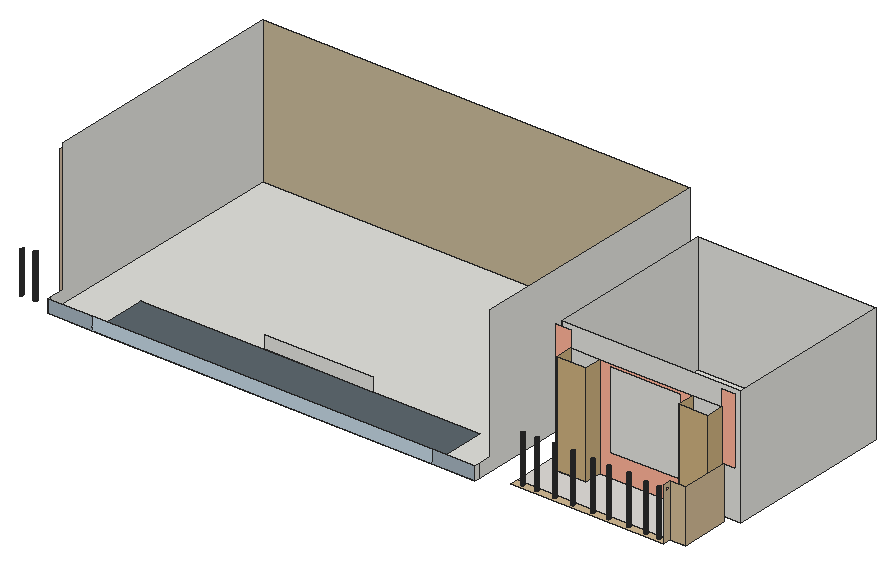
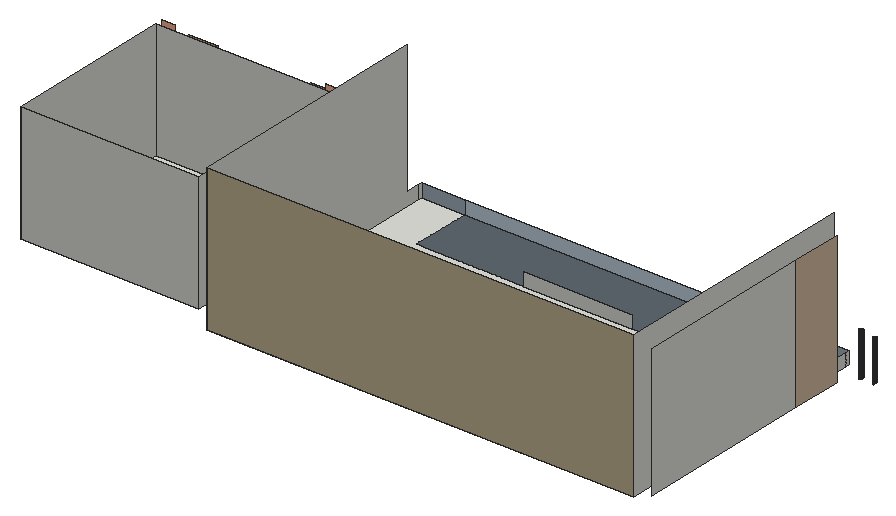
# SketchUp Ruby script. Lengths in inches.
U = 1.inch
M = Sketchup.active_model
def pt(a) = Geom::Point3d.new(a.map { |v| v * U })
def face(e, loops, mat)
  f = e.add_face(loops[0].map { |a| pt(a) })
  loops[1..].each { |l| e.add_face(l.map { |a| pt(a) }).erase! }
  f.material = f.back_material = mat if mat
  f
end
# faces: each face lists its corners as indices into pts; further lists are holes
def faces(e, pts, list, mat = nil) = list.each { |f| face(e, (f[0].is_a?(Array) ? f : [f]).map { |l| l.map { |i| pts[i] } }, mat) }
# xy, xz, yz: faces in a plane at the given z, y or x. An outline is a flat list of corners, or four numbers for a rectangle; further outlines are holes
def ring(l) = l.size == 4 ? [[l[0], l[1]], [l[2], l[1]], [l[2], l[3]], [l[0], l[3]]] : l.each_slice(2).to_a
def flat(e, list, mat, &to3) = list.each { |f| face(e, (f[0].is_a?(Array) ? f : [f]).map { |l| ring(l).map { |u, v| to3.(u, v) } }, mat) }
def xy(e, z, list, mat = nil) = flat(e, list, mat) { |x, y| [x, y, z] }
def xz(e, y, list, mat = nil) = flat(e, list, mat) { |x, z| [x, y, z] }
def yz(e, x, list, mat = nil) = flat(e, list, mat) { |y, z| [x, y, z] }
def lines(e, pts, list) = list.each { |a, b| e.add_line(pt(pts[a]), pt(pts[b])) }
# prism: a flat outline (further loops are holes) pulled along v
def prism(e, loops, v, mat = nil)
  f = face(e, loops, mat); d = Geom::Vector3d.new(v.map { |x| x * U })
  f.pushpull(f.normal.samedirection?(d) ? d.length : -d.length)
end
def box(e, o, s, mat = nil) = prism(e, [[o, [o[0] + s[0], o[1], o[2]], [o[0] + s[0], o[1] + s[1], o[2]], [o[0], o[1] + s[1], o[2]]]], [0, 0, s[2]], mat)
def at(x, y, z, deg = 0) = Geom::Transformation.translation(pt([x, y, z])) * Geom::Transformation.rotation(ORIGIN, Z_AXIS, deg.degrees)
def axes(o, x, y, z) = Geom::Transformation.new([*x, 0, *y, 0, *z, 0, *pt(o).to_a, 1])
def part(name) = M.definitions.add(name)
# library, detail: a bought-in or finely detailed component or shape, given as its bounding box
def library(name, o, s) = part(name).tap { |d| box(d.entities, o, s) }
def detail(e, o, s) = box(e.add_group.entities, o, s)
def put(e, d, t, mat = nil) = e.add_instance(d, t).tap { |i| i.material = mat if mat }
def group(e, t, mat = nil) = e.add_group.tap { |g| g.transformation = t; g.material = mat if mat }.entities
root = M.entities
M.materials.add("[Color B02]").color = [255, 178, 153]
M.materials.add("[Formica Beige]").color = [211, 187, 149]
M.materials.add("[Formica Laminate Dark]").color = [50, 53, 60]
M.materials.add("[Formica Laminate Light]").color = [213, 189, 164]
M.materials.add("[Formica Speckled Grey]").color = [94, 105, 111]
M.materials.add("[Quartz Light Brown]").color = [199, 184, 152]
M.materials.add("[Terrazzo Light Blue]1").color = [165, 180, 191]
M.materials.add("[Terrazzo Light Blue]2").color = [196, 214, 227]
M.materials.add("[Terrazzo Tile Accent]").color = [224, 221, 217]
M.materials.add("[Wood Floor Light]").color = [204, 176, 127]
xy(root,381,[[198.57,119.07,198.57,364.125,588.3,364.125,588.3,119.07,549.2,119.07,549.2,174.4375,238.58,174.4375,238.58,119.07],[179.57,126.78,179.17,126.87,178.8125,127.0625,178.51,127.34,178.3,127.6875,178.18,128.08,178.17,128.48,178.26,128.88,178.45,129.24,178.73,129.54,179.07,129.76,179.46,129.875,179.87,129.89,180.27,129.8,180.63,129.6,180.93,129.33,181.14,128.98,181.26,128.59,181.28,128.18,181.18,127.78,180.99,127.42,180.71,127.125,180.37,126.91,179.98,126.79],[618.46,134.27,618.09,134.32,617.75,134.46,617.45,134.6875,617.22,134.99,617.08,135.33,617.03,135.7,617.08,136.08,617.22,136.42,617.45,136.72,617.75,136.95,618.09,137.09,618.46,137.14,618.84,137.09,619.18,136.95,619.48,136.72,619.71,136.42,619.85,136.08,619.9,135.7,619.85,135.33,619.71,134.99,619.48,134.6875,619.18,134.46,618.84,134.32],[631.71,134.27,631.34,134.32,631,134.46,630.7,134.6875,630.47,134.99,630.33,135.33,630.28,135.7,630.33,136.08,630.47,136.42,630.7,136.72,631,136.95,631.34,137.09,631.71,137.14,632.09,137.09,632.43,136.95,632.73,136.72,632.96,136.42,633.1,136.08,633.15,135.7,633.1,135.33,632.96,134.99,632.73,134.6875,632.43,134.46,632.09,134.32],[647.4,134.27,647.03,134.32,646.68,134.46,646.39,134.6875,646.16,134.99,646.01,135.33,645.96,135.7,646.01,136.08,646.16,136.42,646.39,136.72,646.68,136.95,647.03,137.09,647.4,137.14,647.77,137.09,648.12,136.95,648.42,136.72,648.65,136.42,648.79,136.08,648.84,135.7,648.79,135.33,648.65,134.99,648.42,134.6875,648.12,134.46,647.77,134.32],
  [664.53,134.27,664.16,134.32,663.81,134.46,663.51,134.6875,663.28,134.99,663.14,135.33,663.09,135.7,663.14,136.08,663.28,136.42,663.51,136.72,663.81,136.95,664.16,137.09,664.53,137.14,664.9,137.09,665.25,136.95,665.54,136.72,665.77,136.42,665.92,136.08,665.96,135.7,665.92,135.33,665.77,134.99,665.54,134.6875,665.25,134.46,664.9,134.32],[682.4,134.27,682.03,134.32,681.68,134.46,681.39,134.6875,681.16,134.99,681.01,135.33,680.96,135.7,681.01,136.08,681.16,136.42,681.39,136.72,681.68,136.95,682.03,137.09,682.4,137.14,682.77,137.09,683.12,136.95,683.42,136.72,683.65,136.42,683.79,136.08,683.84,135.7,683.79,135.33,683.65,134.99,683.42,134.6875,683.12,134.46,682.77,134.32],[697.03,134.27,696.66,134.32,696.31,134.46,696.01,134.6875,695.78,134.99,695.64,135.33,695.59,135.7,695.64,136.08,695.78,136.42,696.01,136.72,696.31,136.95,696.66,137.09,697.03,137.14,697.4,137.09,697.75,136.95,698.04,136.72,698.27,136.42,698.42,136.08,698.46,135.7,698.42,135.33,698.27,134.99,698.04,134.6875,697.75,134.46,697.4,134.32],[715.03,134.27,714.66,134.32,714.31,134.46,714.01,134.6875,713.78,134.99,713.64,135.33,713.59,135.7,713.64,136.08,713.78,136.42,714.01,136.72,714.31,136.95,714.66,137.09,715.03,137.14,715.4,137.09,715.75,136.95,716.04,136.72,716.27,136.42,716.42,136.08,716.46,135.7,716.42,135.33,716.27,134.99,716.04,134.6875,715.75,134.46,715.4,134.32],[730.9,134.27,730.53,134.32,730.18,134.46,729.89,134.6875,729.66,134.99,729.51,135.33,729.46,135.7,729.51,136.08,729.66,136.42,729.89,136.72,730.18,136.95,730.53,137.09,730.9,137.14,731.27,137.09,731.62,136.95,731.92,136.72,732.15,136.42,732.29,136.08,732.34,135.7,732.29,135.33,732.15,134.99,731.92,134.6875,731.62,134.46,731.27,134.32],
  [742.96,134.27,742.59,134.32,742.25,134.46,741.95,134.6875,741.72,134.99,741.58,135.33,741.53,135.7,741.58,136.08,741.72,136.42,741.95,136.72,742.25,136.95,742.59,137.09,742.96,137.14,743.34,137.09,743.68,136.95,743.98,136.72,744.21,136.42,744.35,136.08,744.4,135.7,744.35,135.33,744.21,134.99,743.98,134.6875,743.68,134.46,743.34,134.32],[624.7,167.26,651.04,182.57],[735.89,167.26,762.23,182.57],[611.125,189.24,774.15,344.36]])
xy(root,381,[[[611.125,131.74,750.32,138.95],[742.96,134.27,742.59,134.32,742.25,134.46,741.95,134.6875,741.72,134.99,741.58,135.33,741.53,135.7,741.58,136.08,741.72,136.42,741.95,136.72,742.25,136.95,742.59,137.09,742.96,137.14,743.34,137.09,743.68,136.95,743.98,136.72,744.21,136.42,744.35,136.08,744.4,135.7,744.35,135.33,744.21,134.99,743.98,134.6875,743.68,134.46,743.34,134.32],[618.46,134.27,618.09,134.32,617.75,134.46,617.45,134.6875,617.22,134.99,617.08,135.33,617.03,135.7,617.08,136.08,617.22,136.42,617.45,136.72,617.75,136.95,618.09,137.09,618.46,137.14,618.84,137.09,619.18,136.95,619.48,136.72,619.71,136.42,619.85,136.08,619.9,135.7,619.85,135.33,619.71,134.99,619.48,134.6875,619.18,134.46,618.84,134.32],[730.9,134.27,730.53,134.32,730.18,134.46,729.89,134.6875,729.66,134.99,729.51,135.33,729.46,135.7,729.51,136.08,729.66,136.42,729.89,136.72,730.18,136.95,730.53,137.09,730.9,137.14,731.27,137.09,731.62,136.95,731.92,136.72,732.15,136.42,732.29,136.08,732.34,135.7,732.29,135.33,732.15,134.99,731.92,134.6875,731.62,134.46,731.27,134.32],[631.71,134.27,631.34,134.32,631,134.46,630.7,134.6875,630.47,134.99,630.33,135.33,630.28,135.7,630.33,136.08,630.47,136.42,630.7,136.72,631,136.95,631.34,137.09,631.71,137.14,632.09,137.09,632.43,136.95,632.73,136.72,632.96,136.42,633.1,136.08,633.15,135.7,633.1,135.33,632.96,134.99,632.73,134.6875,632.43,134.46,632.09,134.32],[715.03,134.27,714.66,134.32,714.31,134.46,714.01,134.6875,713.78,134.99,713.64,135.33,713.59,135.7,713.64,136.08,713.78,136.42,714.01,136.72,714.31,136.95,714.66,137.09,715.03,137.14,715.4,137.09,715.75,136.95,716.04,136.72,716.27,136.42,716.42,136.08,716.46,135.7,716.42,135.33,716.27,134.99,716.04,134.6875,715.75,134.46,715.4,134.32],[647.4,134.27,647.03,134.32,646.68,134.46,646.39,134.6875,646.16,134.99,646.01,135.33,645.96,135.7,646.01,136.08,646.16,136.42,646.39,136.72,646.68,136.95,647.03,137.09,647.4,137.14,647.77,137.09,648.12,136.95,648.42,136.72,648.65,136.42,648.79,136.08,648.84,135.7,648.79,135.33,648.65,134.99,648.42,134.6875,648.12,134.46,647.77,134.32],[697.03,134.27,696.66,134.32,696.31,134.46,696.01,134.6875,695.78,134.99,695.64,135.33,695.59,135.7,695.64,136.08,695.78,136.42,696.01,136.72,696.31,136.95,696.66,137.09,697.03,137.14,697.4,137.09,697.75,136.95,698.04,136.72,698.27,136.42,698.42,136.08,698.46,135.7,698.42,135.33,698.27,134.99,698.04,134.6875,697.75,134.46,697.4,134.32],[664.53,134.27,664.16,134.32,663.81,134.46,663.51,134.6875,663.28,134.99,663.14,135.33,663.09,135.7,663.14,136.08,663.28,136.42,663.51,136.72,663.81,136.95,664.16,137.09,664.53,137.14,664.9,137.09,665.25,136.95,665.54,136.72,665.77,136.42,665.92,136.08,665.96,135.7,665.92,135.33,665.77,134.99,665.54,134.6875,665.25,134.46,664.9,134.32],[682.4,134.27,682.03,134.32,681.68,134.46,681.39,134.6875,681.16,134.99,681.01,135.33,680.96,135.7,681.01,136.08,681.16,136.42,681.39,136.72,681.68,136.95,682.03,137.09,682.4,137.14,682.77,137.09,683.12,136.95,683.42,136.72,683.65,136.42,683.79,136.08,683.84,135.7,683.79,135.33,683.65,134.99,683.42,134.6875,683.12,134.46,682.77,134.32]]],"[Formica Beige]")
xy(root,381,[[238.58,119.07,549.2,174.4375]],"[Formica Speckled Grey]")
xy(root,381,[[611.125,138.95,764.43,138.95,764.43,182.57,762.23,182.57,762.23,167.26,735.89,167.26,735.89,182.57,651.04,182.57,651.04,167.26,624.7,167.26,624.7,182.57,611.125,182.57]],"[Terrazzo Tile Accent]")
xz(root,119.07,[[198.57,381,238.58,393],[549.2,381,588.3,393]],"[Terrazzo Light Blue]1")
xz(root,119.07,[[238.58,381,549.2,393]],"[Terrazzo Light Blue]2")
xz(root,138.95,[[750.32,381,764.43,429]],"[Formica Beige]")
xz(root,167.26,[[624.7,381,651.04,474.11],[735.89,381,762.23,474.11]],"[Wood Floor Light]")
xz(root,174.4375,[[351.88,381,450.54,393]])
xz(root,182.57,[[624.7,381,651.04,474.11],[735.89,381,762.23,474.11]])
xz(root,182.57,[[611.125,381,624.7,489],[[651.04,381,735.89,474.11],[660.63,401.51,725.25,472.38]],[762.23,381,764.43,381,764.43,429,774.15,429,774.15,489,762.23,489]],"[Color B02]")
xz(root,189.24,[[611.125,381,774.15,489]])
xz(root,344.36,[[611.125,381,774.15,489]])
xz(root,364.125,[[198.57,381,588.3,513]],"[Quartz Light Brown]")
yz(root,189.57,[[191.15,381,355.125,501]])
yz(root,189.57,[[144.21,381,191.15,501]],"[Formica Laminate Light]")
yz(root,198.57,[[119.07,381,122.79,393],[122.79,381,122.79,393,135.71,393,135.71,513,364.125,513,364.125,381]])
yz(root,588.3,[[119.07,381,122.79,393],[122.79,381,122.79,393,135.71,393,135.71,513,364.125,513,364.125,381]])
yz(root,611.125,[[189.24,381,344.36,489]])
yz(root,624.7,[[167.26,381,182.57,474.11]],"[Wood Floor Light]")
yz(root,651.04,[[167.26,381,182.57,474.11]],"[Wood Floor Light]")
yz(root,735.89,[[167.26,381,182.57,474.11]],"[Wood Floor Light]")
yz(root,750.32,[[[131.74,381,138.95,429],[135.46,422.23,135.91,422.29,136.33,422.46,136.7,422.74,136.98,423.1,137.15,423.53,137.21,423.98,137.15,424.43,136.98,424.85,136.7,425.22,136.33,425.49,135.91,425.67,135.46,425.73,135.01,425.67,134.58,425.49,134.22,425.22,133.94,424.85,133.77,424.43,133.71,423.98,133.77,423.53,133.94,423.1,134.22,422.74,134.58,422.46,135.01,422.29]]],"[Formica Beige]")
yz(root,762.23,[[167.26,381,182.57,474.11]],"[Wood Floor Light]")
yz(root,764.43,[[138.95,381,182.57,429]],"[Formica Beige]")
yz(root,774.15,[[189.24,381,344.36,489]])
p = [[167.1,126.79,381],[167.49,126.91,381],[167.49,126.91,418.875],[167.1,126.79,418.875],[179.17,126.87,381],[179.57,126.78,381],
  [179.57,126.78,420.65],[179.17,126.87,420.65],[179.98,126.79,381],[179.98,126.79,420.65],[180.37,126.91,381],[180.37,126.91,420.65],
  [167.84,127.125,381],[167.84,127.125,418.875],[178.8125,127.0625,381],[178.8125,127.0625,420.65],[180.71,127.125,381],[180.71,127.125,420.65],
  [168.12,127.42,381],[168.12,127.42,418.875],[178.51,127.34,381],[178.51,127.34,420.65],[180.99,127.42,381],[180.99,127.42,420.65],
  [178.3,127.6875,381],[178.3,127.6875,420.65],[168.31,127.78,381],[168.31,127.78,418.875],[181.18,127.78,381],[181.18,127.78,420.65],
  [178.18,128.08,381],[178.18,128.08,420.65],[168.4,128.18,381],[168.4,128.18,418.875],[181.28,128.18,381],[181.28,128.18,420.65],
  [178.17,128.48,381],[178.17,128.48,420.65],[168.39,128.59,381],[168.39,128.59,418.875],[181.26,128.59,381],[181.26,128.59,420.65],
  [178.26,128.88,381],[178.26,128.88,420.65],[168.27,128.98,381],[168.27,128.98,418.875],[181.14,128.98,381],[181.14,128.98,420.65],
  [178.45,129.24,381],[178.45,129.24,420.65],[168.05,129.33,381],[168.05,129.33,418.875],[180.93,129.33,381],[180.93,129.33,420.65],
  [178.73,129.54,381],[178.73,129.54,420.65],[167.75,129.6,381],[167.75,129.6,418.875],[180.63,129.6,381],[180.63,129.6,420.65],
  [179.07,129.76,381],[179.07,129.76,420.65],[167.39,129.8,381],[167.39,129.8,418.875],[180.27,129.8,381],[180.27,129.8,420.65],
  [167,129.89,381],[167,129.89,418.875],[179.46,129.875,381],[179.46,129.875,420.65],[179.87,129.89,381],[179.87,129.89,420.65],
  [617.75,134.46,381],[618.09,134.32,381],[618.09,134.32,423.375],[617.75,134.46,423.375],[618.46,134.27,381],[618.46,134.27,423.375],
  [618.84,134.32,381],[618.84,134.32,423.375],[619.18,134.46,381],[619.18,134.46,423.375],[631,134.46,381],[631.34,134.32,381],
  [631.34,134.32,423.6875],[631,134.46,423.6875],[631.71,134.27,381],[631.71,134.27,423.6875],[632.09,134.32,381],[632.09,134.32,423.6875],
  [632.43,134.46,381],[632.43,134.46,423.6875],[646.68,134.46,381],[647.03,134.32,381],[647.03,134.32,424.375],[646.68,134.46,424.375],
  [647.4,134.27,381],[647.4,134.27,424.375],[647.77,134.32,381],[647.77,134.32,424.375],[648.12,134.46,381],[648.12,134.46,424.375],
  [663.81,134.46,381],[664.16,134.32,381],[664.16,134.32,424.8125],[663.81,134.46,424.8125],[664.53,134.27,381],[664.53,134.27,424.8125],
  [664.9,134.32,381],[664.9,134.32,424.8125],[665.25,134.46,381],[665.25,134.46,424.8125],[681.68,134.46,381],[682.03,134.32,381],
  [682.03,134.32,424.25],[681.68,134.46,424.25],[682.4,134.27,381],[682.4,134.27,424.25],[682.77,134.32,381],[682.77,134.32,424.25],
  [683.12,134.46,381],[683.12,134.46,424.25],[696.31,134.46,381],[696.66,134.32,381],[696.66,134.32,423.75],[696.31,134.46,423.75],
  [697.03,134.27,381],[697.03,134.27,423.75],[697.4,134.32,381],[697.4,134.32,423.75],[697.75,134.46,381],[697.75,134.46,423.75],
  [714.31,134.46,381],[714.66,134.32,381],[714.66,134.32,424.43],[714.31,134.46,424.43],[715.03,134.27,381],[715.03,134.27,424.43],
  [715.4,134.32,381],[715.4,134.32,424.43],[715.75,134.46,381],[715.75,134.46,424.43],[730.18,134.46,381],[730.53,134.32,381],
  [730.53,134.32,422.625],[730.18,134.46,422.625],[730.9,134.27,381],[730.9,134.27,422.625],[731.27,134.32,381],[731.27,134.32,422.625],
  [731.62,134.46,381],[731.62,134.46,422.625],[742.25,134.46,381],[742.59,134.32,381],[742.59,134.32,423.0625],[742.25,134.46,423.0625],
  [742.96,134.27,381],[742.96,134.27,423.0625],[743.34,134.32,381],[743.34,134.32,423.0625],[743.68,134.46,381],[743.68,134.46,423.0625],
  [617.45,134.6875,381],[617.45,134.6875,423.375],[619.48,134.6875,381],[619.48,134.6875,423.375],[630.7,134.6875,381],[630.7,134.6875,423.6875],
  [632.73,134.6875,381],[632.73,134.6875,423.6875],[646.39,134.6875,381],[646.39,134.6875,424.375],[648.42,134.6875,381],[648.42,134.6875,424.375],
  [663.51,134.6875,381],[663.51,134.6875,424.8125],[665.54,134.6875,381],[665.54,134.6875,424.8125],[681.39,134.6875,381],[681.39,134.6875,424.25],
  [683.42,134.6875,381],[683.42,134.6875,424.25],[696.01,134.6875,381],[696.01,134.6875,423.75],[698.04,134.6875,381],[698.04,134.6875,423.75],
  [714.01,134.6875,381],[714.01,134.6875,424.43],[716.04,134.6875,381],[716.04,134.6875,424.43],[729.89,134.6875,381],[729.89,134.6875,422.625],
  [731.92,134.6875,381],[731.92,134.6875,422.625],[741.95,134.6875,381],[741.95,134.6875,423.0625],[743.98,134.6875,381],[743.98,134.6875,423.0625],
  [617.22,134.99,381],[617.22,134.99,423.375],[619.71,134.99,381],[619.71,134.99,423.375],[630.47,134.99,381],[630.47,134.99,423.6875],
  [632.96,134.99,381],[632.96,134.99,423.6875],[646.16,134.99,381],[646.16,134.99,424.375],[648.65,134.99,381],[648.65,134.99,424.375],
  [663.28,134.99,381],[663.28,134.99,424.8125],[665.77,134.99,381],[665.77,134.99,424.8125],[681.16,134.99,381],[681.16,134.99,424.25],
  [683.65,134.99,381],[683.65,134.99,424.25],[695.78,134.99,381],[695.78,134.99,423.75],[698.27,134.99,381],[698.27,134.99,423.75],
  [713.78,134.99,381],[713.78,134.99,424.43],[716.27,134.99,381],[716.27,134.99,424.43],[729.66,134.99,381],[729.66,134.99,422.625],
  [732.15,134.99,381],[732.15,134.99,422.625],[741.72,134.99,381],[741.72,134.99,423.0625],[744.21,134.99,381],[744.21,134.99,423.0625],
  [617.08,135.33,381],[617.08,135.33,423.375],[619.85,135.33,381],[619.85,135.33,423.375],[630.33,135.33,381],[630.33,135.33,423.6875],
  [633.1,135.33,381],[633.1,135.33,423.6875],[646.01,135.33,381],[646.01,135.33,424.375],[648.79,135.33,381],[648.79,135.33,424.375],
  [663.14,135.33,381],[663.14,135.33,424.8125],[665.92,135.33,381],[665.92,135.33,424.8125],[681.01,135.33,381],[681.01,135.33,424.25],
  [683.79,135.33,381],[683.79,135.33,424.25],[695.64,135.33,381],[695.64,135.33,423.75],[698.42,135.33,381],[698.42,135.33,423.75],
  [713.64,135.33,381],[713.64,135.33,424.43],[716.42,135.33,381],[716.42,135.33,424.43],[729.51,135.33,381],[729.51,135.33,422.625],
  [732.29,135.33,381],[732.29,135.33,422.625],[741.58,135.33,381],[741.58,135.33,423.0625],[744.35,135.33,381],[744.35,135.33,423.0625],
  [617.03,135.7,381],[617.03,135.7,423.375],[619.9,135.7,381],[619.9,135.7,423.375],[630.28,135.7,381],[630.28,135.7,423.6875],
  [633.15,135.7,381],[633.15,135.7,423.6875],[645.96,135.7,381],[645.96,135.7,424.375],[648.84,135.7,381],[648.84,135.7,424.375],
  [663.09,135.7,381],[663.09,135.7,424.8125],[665.96,135.7,381],[665.96,135.7,424.8125],[680.96,135.7,381],[680.96,135.7,424.25],
  [683.84,135.7,381],[683.84,135.7,424.25],[695.59,135.7,381],[695.59,135.7,423.75],[698.46,135.7,381],[698.46,135.7,423.75],
  [713.59,135.7,381],[713.59,135.7,424.43],[716.46,135.7,381],[716.46,135.7,424.43],[729.46,135.7,381],[729.46,135.7,422.625],
  [732.34,135.7,381],[732.34,135.7,422.625],[741.53,135.7,381],[741.53,135.7,423.0625],[744.4,135.7,381],[744.4,135.7,423.0625],
  [617.08,136.08,381],[617.08,136.08,423.375],[619.85,136.08,381],[619.85,136.08,423.375],[630.33,136.08,381],[630.33,136.08,423.6875],
  [633.1,136.08,381],[633.1,136.08,423.6875],[646.01,136.08,381],[646.01,136.08,424.375],[648.79,136.08,381],[648.79,136.08,424.375],
  [663.14,136.08,381],[663.14,136.08,424.8125],[665.92,136.08,381],[665.92,136.08,424.8125],[681.01,136.08,381],[681.01,136.08,424.25],
  [683.79,136.08,381],[683.79,136.08,424.25],[695.64,136.08,381],[695.64,136.08,423.75],[698.42,136.08,381],[698.42,136.08,423.75],
  [713.64,136.08,381],[713.64,136.08,424.43],[716.42,136.08,381],[716.42,136.08,424.43],[729.51,136.08,381],[729.51,136.08,422.625],
  [732.29,136.08,381],[732.29,136.08,422.625],[741.58,136.08,381],[741.58,136.08,423.0625],[744.35,136.08,381],[744.35,136.08,423.0625],
  [617.22,136.42,381],[617.22,136.42,423.375],[619.71,136.42,381],[619.71,136.42,423.375],[630.47,136.42,381],[630.47,136.42,423.6875],
  [632.96,136.42,381],[632.96,136.42,423.6875],[646.16,136.42,381],[646.16,136.42,424.375],[648.65,136.42,381],[648.65,136.42,424.375],
  [663.28,136.42,381],[663.28,136.42,424.8125],[665.77,136.42,381],[665.77,136.42,424.8125],[681.16,136.42,381],[681.16,136.42,424.25],
  [683.65,136.42,381],[683.65,136.42,424.25],[695.78,136.42,381],[695.78,136.42,423.75],[698.27,136.42,381],[698.27,136.42,423.75],
  [713.78,136.42,381],[713.78,136.42,424.43],[716.27,136.42,381],[716.27,136.42,424.43],[729.66,136.42,381],[729.66,136.42,422.625],
  [732.15,136.42,381],[732.15,136.42,422.625],[741.72,136.42,381],[741.72,136.42,423.0625],[744.21,136.42,381],[744.21,136.42,423.0625],
  [617.45,136.72,381],[617.45,136.72,423.375],[619.48,136.72,381],[619.48,136.72,423.375],[630.7,136.72,381],[630.7,136.72,423.6875],
  [632.73,136.72,381],[632.73,136.72,423.6875],[646.39,136.72,381],[646.39,136.72,424.375],[648.42,136.72,381],[648.42,136.72,424.375],
  [663.51,136.72,381],[663.51,136.72,424.8125],[665.54,136.72,381],[665.54,136.72,424.8125],[681.39,136.72,381],[681.39,136.72,424.25],
  [683.42,136.72,381],[683.42,136.72,424.25],[696.01,136.72,381],[696.01,136.72,423.75],[698.04,136.72,381],[698.04,136.72,423.75],
  [714.01,136.72,381],[714.01,136.72,424.43],[716.04,136.72,381],[716.04,136.72,424.43],[729.89,136.72,381],[729.89,136.72,422.625],
  [731.92,136.72,381],[731.92,136.72,422.625],[741.95,136.72,381],[741.95,136.72,423.0625],[743.98,136.72,381],[743.98,136.72,423.0625],
  [617.75,136.95,381],[617.75,136.95,423.375],[619.18,136.95,381],[619.18,136.95,423.375],[631,136.95,381],[631,136.95,423.6875],
  [632.43,136.95,381],[632.43,136.95,423.6875],[646.68,136.95,381],[646.68,136.95,424.375],[648.12,136.95,381],[648.12,136.95,424.375],
  [663.81,136.95,381],[663.81,136.95,424.8125],[665.25,136.95,381],[665.25,136.95,424.8125],[681.68,136.95,381],[681.68,136.95,424.25],
  [683.12,136.95,381],[683.12,136.95,424.25],[696.31,136.95,381],[696.31,136.95,423.75],[697.75,136.95,381],[697.75,136.95,423.75],
  [714.31,136.95,381],[714.31,136.95,424.43],[715.75,136.95,381],[715.75,136.95,424.43],[730.18,136.95,381],[730.18,136.95,422.625],
  [731.62,136.95,381],[731.62,136.95,422.625],[742.25,136.95,381],[742.25,136.95,423.0625],[743.68,136.95,381],[743.68,136.95,423.0625],
  [618.09,137.09,381],[618.09,137.09,423.375],[618.84,137.09,381],[618.84,137.09,423.375],[631.34,137.09,381],[631.34,137.09,423.6875],
  [632.09,137.09,381],[632.09,137.09,423.6875],[647.03,137.09,381],[647.03,137.09,424.375],[647.77,137.09,381],[647.77,137.09,424.375],
  [664.16,137.09,381],[664.16,137.09,424.8125],[664.9,137.09,381],[664.9,137.09,424.8125],[682.03,137.09,381],[682.03,137.09,424.25],
  [682.77,137.09,381],[682.77,137.09,424.25],[696.66,137.09,381],[696.66,137.09,423.75],[697.4,137.09,381],[697.4,137.09,423.75],
  [714.66,137.09,381],[714.66,137.09,424.43],[715.4,137.09,381],[715.4,137.09,424.43],[730.53,137.09,381],[730.53,137.09,422.625],
  [731.27,137.09,381],[731.27,137.09,422.625],[742.59,137.09,381],[742.59,137.09,423.0625],[743.34,137.09,381],[743.34,137.09,423.0625],
  [618.46,137.14,381],[618.46,137.14,423.375],[631.71,137.14,381],[631.71,137.14,423.6875],[647.4,137.14,381],[647.4,137.14,424.375],
  [664.53,137.14,381],[664.53,137.14,424.8125],[682.4,137.14,381],[682.4,137.14,424.25],[697.03,137.14,381],[697.03,137.14,423.75],
  [715.03,137.14,381],[715.03,137.14,424.43],[730.9,137.14,381],[730.9,137.14,422.625],[742.96,137.14,381],[742.96,137.14,423.0625]]
faces(root,p,[[0,1,2,3],[4,5,6,7],[5,8,9,6],[8,10,11,9],[1,12,13,2],[14,4,7,15],[10,16,17,11],[12,18,19,13],
  [20,14,15,21],[16,22,23,17],[24,20,21,25],[18,26,27,19],[22,28,29,23],[30,24,25,31],[26,32,33,27],[28,34,35,29],
  [36,30,31,37],[32,38,39,33],[34,40,41,35],[42,36,37,43],[38,44,45,39],[40,46,47,41],[48,42,43,49],[44,50,51,45],
  [46,52,53,47],[54,48,49,55],[50,56,57,51],[52,58,59,53],[60,54,55,61],[56,62,63,57],[58,64,65,59],[62,66,67,63],
  [68,60,61,69],[64,70,71,65],[70,68,69,71],[72,73,74,75],[73,76,77,74],[76,78,79,77],[78,80,81,79],[82,83,84,85],
  [83,86,87,84],[86,88,89,87],[88,90,91,89],[92,93,94,95],[93,96,97,94],[96,98,99,97],[98,100,101,99],[102,103,104,105],
  [103,106,107,104],[106,108,109,107],[108,110,111,109],[112,113,114,115],[113,116,117,114],[116,118,119,117],[118,120,121,119],[122,123,124,125],
  [123,126,127,124],[126,128,129,127],[128,130,131,129],[132,133,134,135],[133,136,137,134],[136,138,139,137],[138,140,141,139],[142,143,144,145],
  [143,146,147,144],[146,148,149,147],[148,150,151,149],[152,153,154,155],[153,156,157,154],[156,158,159,157],[158,160,161,159],[162,72,75,163],
  [80,164,165,81],[166,82,85,167],[90,168,169,91],[170,92,95,171],[100,172,173,101],[174,102,105,175],[110,176,177,111],[178,112,115,179],
  [120,180,181,121],[182,122,125,183],[130,184,185,131],[186,132,135,187],[140,188,189,141],[190,142,145,191],[150,192,193,151],[194,152,155,195],
  [160,196,197,161],[198,162,163,199],[164,200,201,165],[202,166,167,203],[168,204,205,169],[206,170,171,207],[172,208,209,173],[210,174,175,211],
  [176,212,213,177],[214,178,179,215],[180,216,217,181],[218,182,183,219],[184,220,221,185],[222,186,187,223],[188,224,225,189],[226,190,191,227],
  [192,228,229,193],[230,194,195,231],[196,232,233,197],[234,198,199,235],[200,236,237,201],[238,202,203,239],[204,240,241,205],[242,206,207,243],
  [208,244,245,209],[246,210,211,247],[212,248,249,213],[250,214,215,251],[216,252,253,217],[254,218,219,255],[220,256,257,221],[258,222,223,259],
  [224,260,261,225],[262,226,227,263],[228,264,265,229],[266,230,231,267],[232,268,269,233],[270,234,235,271],[236,272,273,237],[274,238,239,275],
  [240,276,277,241],[278,242,243,279],[244,280,281,245],[282,246,247,283],[248,284,285,249],[286,250,251,287],[252,288,289,253],[290,254,255,291],
  [256,292,293,257],[294,258,259,295],[260,296,297,261],[298,262,263,299],[264,300,301,265],[302,266,267,303],[268,304,305,269],[306,270,271,307],
  [272,308,309,273],[310,274,275,311],[276,312,313,277],[314,278,279,315],[280,316,317,281],[318,282,283,319],[284,320,321,285],[322,286,287,323],
  [288,324,325,289],[326,290,291,327],[292,328,329,293],[330,294,295,331],[296,332,333,297],[334,298,299,335],[300,336,337,301],[338,302,303,339],
  [304,340,341,305],[342,306,307,343],[308,344,345,309],[346,310,311,347],[312,348,349,313],[350,314,315,351],[316,352,353,317],[354,318,319,355],
  [320,356,357,321],[358,322,323,359],[324,360,361,325],[362,326,327,363],[328,364,365,329],[366,330,331,367],[332,368,369,333],[370,334,335,371],
  [336,372,373,337],[374,338,339,375],[340,376,377,341],[378,342,343,379],[344,380,381,345],[382,346,347,383],[348,384,385,349],[386,350,351,387],
  [352,388,389,353],[390,354,355,391],[356,392,393,357],[394,358,359,395],[360,396,397,361],[398,362,363,399],[364,400,401,365],[402,366,367,403],
  [368,404,405,369],[406,370,371,407],[372,408,409,373],[410,374,375,411],[376,412,413,377],[414,378,379,415],[380,416,417,381],[418,382,383,419],
  [384,420,421,385],[422,386,387,423],[388,424,425,389],[426,390,391,427],[392,428,429,393],[430,394,395,431],[396,432,433,397],[434,398,399,435],
  [400,436,437,401],[438,402,403,439],[404,440,441,405],[442,406,407,443],[408,444,445,409],[446,410,411,447],[412,448,449,413],[450,414,415,451],
  [416,452,453,417],[454,418,419,455],[420,456,457,421],[458,422,423,459],[424,460,461,425],[462,426,427,463],[428,464,465,429],[466,430,431,467],
  [432,468,469,433],[470,434,435,471],[436,472,473,437],[474,438,439,475],[440,476,477,441],[478,442,443,479],[444,480,481,445],[482,446,447,483],
  [448,484,485,449],[486,450,451,487],[452,486,487,453],[488,454,455,489],[456,488,489,457],[490,458,459,491],[460,490,491,461],[492,462,463,493],
  [464,492,493,465],[494,466,467,495],[468,494,495,469],[496,470,471,497],[472,496,497,473],[498,474,475,499],[476,498,499,477],[500,478,479,501],
  [480,500,501,481],[502,482,483,503],[484,502,503,485]],"[Formica Laminate Dark]")
